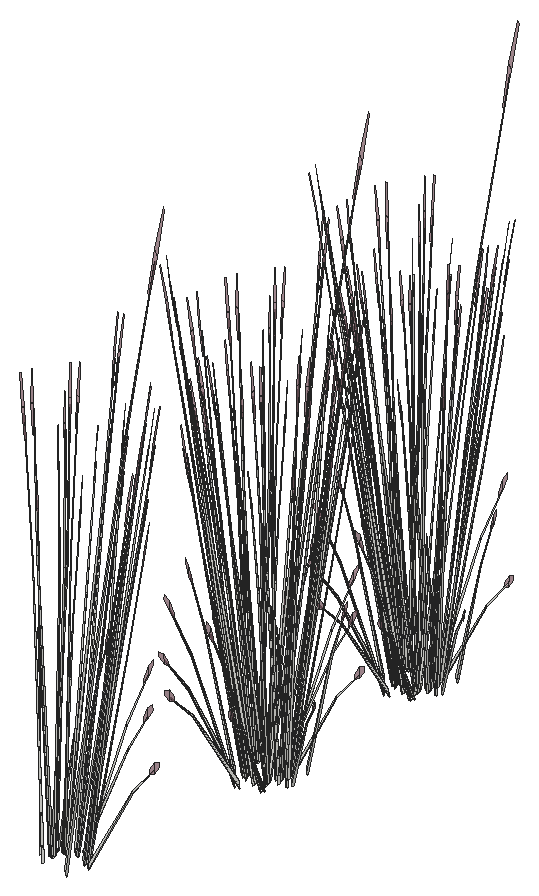
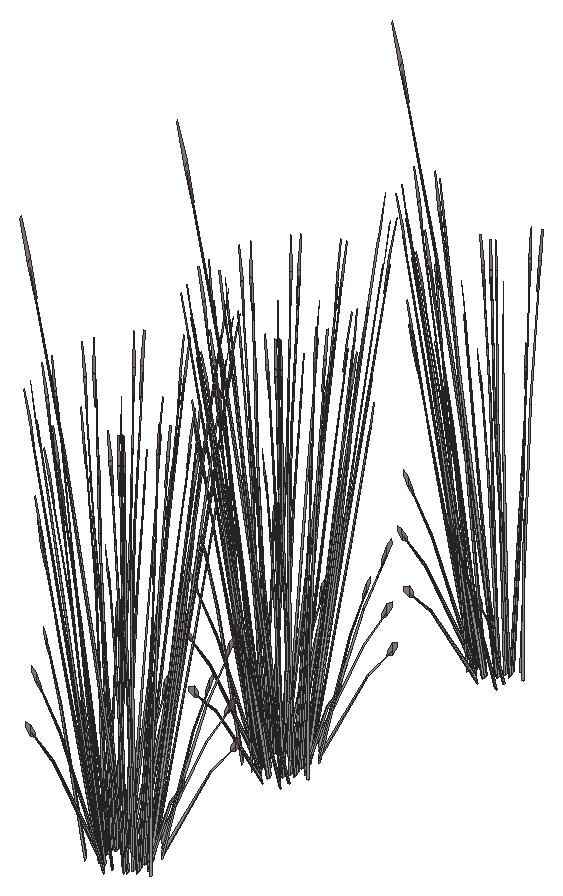
# SketchUp Ruby script. Lengths in inches.
U = 1.inch
M = Sketchup.active_model
def pt(a) = Geom::Point3d.new(a.map { |v| v * U })
def face(e, loops, mat)
  f = e.add_face(loops[0].map { |a| pt(a) })
  loops[1..].each { |l| e.add_face(l.map { |a| pt(a) }).erase! }
  f.material = f.back_material = mat if mat
  f
end
# faces: each face lists its corners as indices into pts; further lists are holes
def faces(e, pts, list, mat = nil) = list.each { |f| face(e, (f[0].is_a?(Array) ? f : [f]).map { |l| l.map { |i| pts[i] } }, mat) }
# xy, xz, yz: faces in a plane at the given z, y or x. An outline is a flat list of corners, or four numbers for a rectangle; further outlines are holes
def ring(l) = l.size == 4 ? [[l[0], l[1]], [l[2], l[1]], [l[2], l[3]], [l[0], l[3]]] : l.each_slice(2).to_a
def flat(e, list, mat, &to3) = list.each { |f| face(e, (f[0].is_a?(Array) ? f : [f]).map { |l| ring(l).map { |u, v| to3.(u, v) } }, mat) }
def xy(e, z, list, mat = nil) = flat(e, list, mat) { |x, y| [x, y, z] }
def xz(e, y, list, mat = nil) = flat(e, list, mat) { |x, z| [x, y, z] }
def yz(e, x, list, mat = nil) = flat(e, list, mat) { |y, z| [x, y, z] }
def lines(e, pts, list) = list.each { |a, b| e.add_line(pt(pts[a]), pt(pts[b])) }
# prism: a flat outline (further loops are holes) pulled along v
def prism(e, loops, v, mat = nil)
  f = face(e, loops, mat); d = Geom::Vector3d.new(v.map { |x| x * U })
  f.pushpull(f.normal.samedirection?(d) ? d.length : -d.length)
end
def box(e, o, s, mat = nil) = prism(e, [[o, [o[0] + s[0], o[1], o[2]], [o[0] + s[0], o[1] + s[1], o[2]], [o[0], o[1] + s[1], o[2]]]], [0, 0, s[2]], mat)
def at(x, y, z, deg = 0) = Geom::Transformation.translation(pt([x, y, z])) * Geom::Transformation.rotation(ORIGIN, Z_AXIS, deg.degrees)
def axes(o, x, y, z) = Geom::Transformation.new([*x, 0, *y, 0, *z, 0, *pt(o).to_a, 1])
def part(name) = M.definitions.add(name)
# library, detail: a bought-in or finely detailed component or shape, given as its bounding box
def library(name, o, s) = part(name).tap { |d| box(d.entities, o, s) }
def detail(e, o, s) = box(e.add_group.entities, o, s)
def put(e, d, t, mat = nil) = e.add_instance(d, t).tap { |i| i.material = mat if mat }
def group(e, t, mat = nil) = e.add_group.tap { |g| g.transformation = t; g.material = mat if mat }.entities
root = M.entities
M.materials.add("LightPink_Translucent").color = [144, 107, 117]
M.materials["LightPink_Translucent"].alpha = 0.75
c1 = part("blade")
p = [[2.15,0.21,22],[0,0.17,0],[0.09,0.45,0],[2.18,0.31,22],[2.29,0.31,22],[0.38,0.45,0],
  [2.48,0.24,33],[2.49,0.24,33],[2.48,0.22,33]]
faces(c1.entities,p,[[0,1,2,3],[4,5,2,3],[6,3,4,7],[8,0,3,6]])
c2 = part("seeds")
p = [[0.3,-0.1,1.38],[-0.01,-0.03,1.59],[-0.01,-0.03,0.03],[0.14,-0.07,-0.07],[0.29,-0.03,3],[0.15,0.01,3.11]]
faces(c2.entities,p,[[0,1,2,3],[1,0,4,5]],"LightPink_Translucent")
c3 = part("blade with seeds")
put(c3.entities,c1,at(0,0,0))
put(c3.entities,c2,axes([2.4,0.25,30.99],[1.5799,-0.05474,1.17369],[-0.12525,1.92788,0.29478],[-0.07173,-0.02425,1.56792]))
put(root,c3,axes([397.78,218.14,5.03],[0.17758,0.42229,-0.1216],[-0.31518,0.20752,-0.67495],[-0.13282,0.05572,1.02557]))
put(root,c3,axes([400.46,219.96,5.03],[0.0189,-0.47427,-0.1216],[0.35781,0.01296,-0.67495],[0.13781,0.03295,1.02557]))
put(root,c3,axes([400.4,219.78,5.05],[-0.20082,-0.29199,0.35414],[0.2293,-0.2764,-0.4572],[0.1165,0.04206,0.87481]))
put(root,c3,axes([400.77,219.68,4.72],[0.07571,-0.00789,1.74944],[0.20767,-0.36231,-0.27667],[0.13467,0.04783,0.14031]))
put(root,c3,axes([397.74,219.32,4.73],[-0.08753,-0.42921,0.48003],[0.34336,-0.07449,0.3958],[-0.1012,0.10094,0.9933]))
put(root,c3,axes([397.68,219.24,4.73],[-0.2423,-0.19613,0.0643],[0.14107,-0.2793,0.50621],[-0.07768,0.0903,0.77189]))
put(root,c3,axes([397.95,219.18,5.05],[0.30722,-0.06665,0.35414],[0.08112,0.381,-0.4572],[-0.08804,0.10234,0.87481]))
put(root,c3,axes([396.77,219.01,4.71],[0.04504,0.01251,1.77383],[0.13934,0.41205,-0.16761],[-0.0922,0.10815,0.31391]))
put(root,c3,axes([400.59,220.04,4.73],[-0.01777,0.35463,0.0643],[-0.26836,-0.00972,0.50621],[0.1028,0.03711,0.77189]))
put(root,c3,axes([400.61,219.93,4.73],[-0.26024,0.30729,0.48003],[-0.22444,-0.32634,0.3958],[0.1221,0.05668,0.9933]))
put(root,c3,axes([397.26,220.26,5.65],[0.31145,0.12449,-0.06488],[-0.0958,0.38314,-0.29416],[-0.05094,0.05817,0.97024]))
put(root,c3,axes([399.78,220.29,5.05],[-0.05451,-0.37564,0.35414],[0.31161,-0.09919,-0.4572],[0.0837,0.10765,0.87481]))
put(root,c3,axes([399.99,218.125,4.47],[-0.30498,-0.24231,1.38283],[0.32203,-0.37727,0.59665],[0.0984,0.22736,1.33663]))
put(root,c3,axes([397.79,219.15,5.03],[0.32648,0.25715,-0.1216],[-0.18809,0.3724,-0.67495],[-0.09224,0.12945,1.02557]))
put(root,c3,axes([399.75,220.48,5.03],[0.21031,-0.39918,-0.1216],[0.30457,0.22997,-0.67495],[0.10587,0.11278,1.02557]))
put(root,c3,axes([398.37,219.94,5.05],[0.23881,-0.24554,0.35414],[0.22606,0.28036,-0.4572],[-0.0344,0.14245,0.87481]))
put(root,c3,axes([399.48,220.8125,4.71],[0.00104,-0.05646,1.77383],[0.30246,-0.2491,-0.16761],[0.10506,0.08891,0.31391]))
put(root,c3,axes([398.15,220.16,4.73],[-0.29004,-0.02173,0.0643],[0.00795,-0.32812,0.50621],[-0.03035,0.12569,0.77189]))
put(root,c3,axes([398.24,220.19,4.73],[-0.25132,-0.3182,0.48003],[0.2669,-0.27442,0.3958],[-0.04636,0.14929,0.9933]))
put(root,c3,axes([399.04,220.35,5.05],[0.1064,-0.35863,0.35414],[0.31043,0.1046,-0.4572],[0.02846,0.14439,0.87481]))
put(root,c3,axes([399.83,220.625,4.73],[-0.16041,0.29625,0.0643],[-0.22843,-0.17248,0.50621],[0.07385,0.09498,0.77189]))
put(root,c3,axes([399.46,221.625,5.65],[0.2439,-0.26754,-0.06488],[0.22348,0.29302,-0.29416],[0.01573,0.08303,0.97024]))
put(root,c3,axes([399.9,220.54,4.73],[-0.35104,0.10702,0.48003],[-0.06092,-0.41983,0.3958],[0.08256,0.12373,0.9933]))
put(root,c3,axes([398.94,220.67,4.73],[-0.26007,0.1585,0.0643],[-0.12729,-0.28902,0.50621],[0.02512,0.1274,0.77189]))
put(root,c3,axes([397.42,220.22,4.72],[-0.00877,0.09229,1.74944],[0.24897,0.32105,-0.27667],[-0.06518,0.15182,0.14031]))
put(root,c3,axes([398.22,220.01,5.4],[0.3879,0.02311,-0.13498],[-0.0106,0.43749,-0.74919],[-0.02694,0.1685,1.13838]))
put(root,c3,axes([398.93,220.5,5.03],[0.34538,-0.21713,-0.1216],[0.16972,0.38536,-0.67495],[0.04557,0.16239,1.02557]))
put(root,c3,axes([399.03,220.64,5.0625],[-0.34777,-0.12192,0.53283],[0.11892,-0.40083,0.43934],[0.0209,0.15763,1.10256]))
put(root,c3,axes([397.39,221.16,4.71],[0.04004,-0.02816,1.77383],[0.33095,0.18728,-0.16761],[-0.00778,0.15594,0.31391]))
put(root,c3,axes([398.85,221.36,4.72],[0.04474,0.0751,1.74944],[0.36104,0.0295,-0.27667],[0.03631,0.16562,0.14031]))
put(root,c3,axes([401.89,235.44,4.72],[-0.05398,-0.06539,1.74944],[-0.36026,0.04145,-0.27667],[-0.0575,-0.15639,0.14031]))
put(root,c3,axes([403.51,236.24,4.72],[-0.00341,-0.09282,1.74944],[-0.28775,-0.26825,-0.27667],[0.04449,-0.16261,0.14031]))
put(root,c3,axes([403.43,235.91,4.71],[-0.03584,0.03562,1.77383],[-0.35118,-0.12018,-0.16761],[-0.01271,-0.15545,0.31391]))
put(root,c3,axes([401.52,235.23,4.71],[-0.00658,0.0559,1.77383],[-0.32474,0.20287,-0.16761],[-0.09556,-0.1037,0.31391]))
put(root,c3,axes([401.45,236.22,5.09],[0.39316,-0.11987,0.53763],[0.06823,0.47021,0.4433],[-0.09247,-0.13858,1.11249]))
put(root,c3,axes([402.34,236.31,4.73],[0.34777,0.12192,0.48003],[-0.11892,0.40083,0.3958],[-0.0209,-0.15763,0.9933]))
put(root,c3,axes([402.4375,236.45,5.03],[-0.34538,0.21713,-0.1216],[-0.16972,-0.38536,-0.67495],[-0.04557,-0.16239,1.02557]))
put(root,c3,axes([403.15,236.9375,5.03],[-0.3879,-0.02311,-0.1216],[0.0106,-0.43749,-0.67495],[0.02694,-0.1685,1.02557]))
put(root,c3,axes([402.43,236.28,4.73],[0.26007,-0.1585,0.0643],[0.12729,0.28902,0.50621],[-0.02512,-0.1274,0.77189]))
put(root,c3,axes([401.54,236.32,4.73],[0.16041,-0.29625,0.0643],[0.22843,0.17248,0.50621],[-0.07385,-0.09498,0.77189]))
put(root,c3,axes([402.33,236.6,5.05],[-0.1064,0.35863,0.35414],[-0.31043,-0.1046,-0.4572],[-0.02846,-0.14439,0.87481]))
put(root,c3,axes([403.125,236.75,4.73],[0.25132,0.3182,0.48003],[-0.2669,0.27442,0.3958],[0.04636,-0.14929,0.9933]))
put(root,c3,axes([401.61,236.29,5.43],[-0.23555,0.44708,-0.13619],[-0.34112,-0.25757,-0.75594],[-0.11858,-0.12631,1.14864]))
put(root,c3,axes([403.22,236.78,4.73],[0.29004,0.02173,0.0643],[-0.00795,0.32812,0.50621],[0.03035,-0.12569,0.77189]))
put(root,c3,axes([403,237.01,5.05],[-0.23881,0.24554,0.35414],[-0.22606,-0.28036,-0.4572],[0.0344,-0.14245,0.87481]))
put(root,c3,axes([400.71,236.16,4.72],[-0.07594,-0.00329,1.74944],[-0.24177,0.32918,-0.27667],[-0.129,-0.06726,0.14031]))
put(root,c3,axes([403.58,237.8,5.03],[-0.32648,-0.25715,-0.1216],[0.18809,-0.3724,-0.67495],[0.09224,-0.12945,1.02557]))
put(root,c3,axes([401.59,236.66,5.05],[0.05451,0.37564,0.35414],[-0.31161,0.09919,-0.4572],[-0.0837,-0.10765,0.87481]))
put(root,c3,axes([400.65,236.91,5.09],[0.29147,-0.34417,0.53763],[0.25138,0.3655,0.4433],[-0.13675,-0.06349,1.11249]))
put(root,c3,axes([404.38,237.6875,4.71],[-0.0461,-0.00354,1.77383],[-0.19143,-0.37951,-0.16761],[0.07688,-0.12478,0.31391]))
put(root,c3,axes([400.78,236.9,4.73],[0.01777,-0.35463,0.0643],[0.26836,0.00972,0.50621],[-0.1028,-0.03711,0.77189]))
put(root,c3,axes([403.42,237.76,5.05],[-0.30722,0.06665,0.35414],[-0.08112,-0.381,-0.4572],[0.08804,-0.10234,0.87481]))
put(root,c3,axes([403.7,237.7,4.73],[0.2423,0.19613,0.0643],[-0.14107,0.2793,0.50621],[0.07768,-0.0903,0.77189]))
put(root,c3,axes([403.63,237.62,4.73],[0.08753,0.42921,0.48003],[-0.34336,0.07449,0.3958],[0.1012,-0.10094,0.9933]))
put(root,c3,axes([404.55,238.14,4.72],[0.04898,-0.07104,1.74944],[-0.06269,-0.43574,-0.27667],[0.12289,-0.08262,0.14031]))
put(root,c3,axes([400.42,236.44,4.71],[0.02617,0.04654,1.77383],[-0.12614,0.41836,-0.16761],[-0.12775,0.00303,0.31391]))
put(root,c3,axes([400.97,237.17,5.05],[0.20082,0.29199,0.35414],[-0.2293,0.2764,-0.4572],[-0.1165,-0.04206,0.87481]))
put(root,c3,axes([400.91,236.98,5.03],[-0.0189,0.47427,-0.1216],[-0.35781,-0.01296,-0.67495],[-0.13781,-0.03295,1.02557]))
put(root,c3,axes([403.59,238.8,5.03],[-0.17758,-0.42229,-0.1216],[0.31518,-0.20752,-0.67495],[0.13282,-0.05572,1.02557]))
put(root,c3,axes([403.47,238.68,5.05],[-0.29332,-0.1301,0.35414],[0.08555,-0.37955,-0.4572],[0.11809,-0.0348,0.87481]))
put(root,c3,axes([400.4,237.98,4.73],[0.09971,-0.42522,0.48003],[0.32782,0.1454,0.3958],[-0.12892,0.02555,0.9933]))
put(root,c3,axes([400.37,237.87,4.73],[-0.12963,-0.31798,0.0643],[0.23638,-0.15564,0.50621],[-0.1042,0.03071,0.77189]))
put(root,c3,axes([403.73,238.79,4.73],[0.12963,0.31798,0.0643],[-0.23638,0.15564,0.50621],[0.1042,-0.03071,0.77189]))
put(root,c3,axes([403.71,238.68,4.73],[-0.09971,0.42522,0.48003],[-0.32782,-0.1454,0.3958],[0.12892,-0.02555,0.9933]))
put(root,c3,axes([400.64,237.99,5.05],[0.29332,0.1301,0.35414],[-0.08555,0.37955,-0.4572],[-0.11809,0.0348,0.87481]))
put(root,c3,axes([404.3,240.06,4.71],[-0.03191,-0.04083,1.77383],[0.06981,-0.43764,-0.16761],[0.12571,-0.02796,0.31391]))
put(root,c3,axes([400.14,238.28,4.72],[-0.05763,0.06055,1.74944],[0.0049,0.44239,-0.27667],[-0.13211,0.05753,0.14031]))
put(root,c3,axes([400.51,237.86,5.03],[0.17758,0.42229,-0.1216],[-0.31518,0.20752,-0.67495],[-0.13282,0.05572,1.02557]))
put(root,c3,axes([403.19,239.68,5.03],[0.0189,-0.47427,-0.1216],[0.35781,0.01296,-0.67495],[0.13781,0.03295,1.02557]))
put(root,c3,axes([403.14,239.49,5.05],[-0.20082,-0.29199,0.35414],[0.2293,-0.2764,-0.4572],[0.1165,0.04206,0.87481]))
put(root,c3,axes([403.5,239.4,4.72],[0.07571,-0.00789,1.74944],[0.20767,-0.36231,-0.27667],[0.13467,0.04783,0.14031]))
put(root,c3,axes([400.47,239.04,4.73],[-0.08753,-0.42921,0.48003],[0.34336,-0.07449,0.3958],[-0.1012,0.10094,0.9933]))
put(root,c3,axes([400.41,238.96,4.73],[-0.2423,-0.19613,0.0643],[0.14107,-0.2793,0.50621],[-0.07768,0.0903,0.77189]))
put(root,c3,axes([400.6875,238.9,5.05],[0.30722,-0.06665,0.35414],[0.08112,0.381,-0.4572],[-0.08804,0.10234,0.87481]))
put(root,c3,axes([399.5,238.73,4.71],[0.04504,0.01251,1.77383],[0.13934,0.41205,-0.16761],[-0.0922,0.10815,0.31391]))
put(root,c3,axes([403.32,239.76,4.73],[-0.01777,0.35463,0.0643],[-0.26836,-0.00972,0.50621],[0.1028,0.03711,0.77189]))
put(root,c3,axes([403.34,239.65,4.73],[-0.26024,0.30729,0.48003],[-0.22444,-0.32634,0.3958],[0.1221,0.05668,0.9933]))
put(root,c3,axes([399.99,239.98,5.65],[0.31145,0.12449,-0.06488],[-0.0958,0.38314,-0.29416],[-0.05094,0.05817,0.97024]))
put(root,c3,axes([402.52,240,5.05],[-0.05451,-0.37564,0.35414],[0.31161,-0.09919,-0.4572],[0.0837,0.10765,0.87481]))
put(root,c3,axes([402.72,237.84,4.47],[-0.30498,-0.24231,1.38283],[0.32203,-0.37727,0.59665],[0.0984,0.22736,1.33663]))
put(root,c3,axes([400.53,238.86,5.03],[0.32648,0.25715,-0.1216],[-0.18809,0.3724,-0.67495],[-0.09224,0.12945,1.02557]))
put(root,c3,axes([402.49,240.2,5.03],[0.21031,-0.39918,-0.1216],[0.30457,0.22997,-0.67495],[0.10587,0.11278,1.02557]))
put(root,c3,axes([401.1,239.66,5.05],[0.23881,-0.24554,0.35414],[0.22606,0.28036,-0.4572],[-0.0344,0.14245,0.87481]))
put(root,c3,axes([402.21,240.53,4.71],[0.00104,-0.05646,1.77383],[0.30246,-0.2491,-0.16761],[0.10506,0.08891,0.31391]))
put(root,c3,axes([400.88,239.88,4.73],[-0.29004,-0.02173,0.0643],[0.00795,-0.32812,0.50621],[-0.03035,0.12569,0.77189]))
put(root,c3,axes([400.98,239.91,4.73],[-0.25132,-0.3182,0.48003],[0.2669,-0.27442,0.3958],[-0.04636,0.14929,0.9933]))
put(root,c3,axes([401.77,240.0625,5.05],[0.1064,-0.35863,0.35414],[0.31043,0.1046,-0.4572],[0.02846,0.14439,0.87481]))
put(root,c3,axes([402.56,240.34,4.73],[-0.16041,0.29625,0.0643],[-0.22843,-0.17248,0.50621],[0.07385,0.09498,0.77189]))
put(root,c3,axes([402.1875,241.34,5.65],[0.2439,-0.26754,-0.06488],[0.22348,0.29302,-0.29416],[0.01573,0.08303,0.97024]))
put(root,c3,axes([402.63,240.26,4.73],[-0.35104,0.10702,0.48003],[-0.06092,-0.41983,0.3958],[0.08256,0.12373,0.9933]))
put(root,c3,axes([401.67,240.39,4.73],[-0.26007,0.1585,0.0643],[-0.12729,-0.28902,0.50621],[0.02512,0.1274,0.77189]))
put(root,c3,axes([400.15,239.93,4.72],[-0.00877,0.09229,1.74944],[0.24897,0.32105,-0.27667],[-0.06518,0.15182,0.14031]))
put(root,c3,axes([400.95,239.72,5.4],[0.3879,0.02311,-0.13498],[-0.0106,0.43749,-0.74919],[-0.02694,0.1685,1.13838]))
put(root,c3,axes([401.67,240.21,5.03],[0.34538,-0.21713,-0.1216],[0.16972,0.38536,-0.67495],[0.04557,0.16239,1.02557]))
put(root,c3,axes([401.77,240.36,5.0625],[-0.34777,-0.12192,0.53283],[0.11892,-0.40083,0.43934],[0.0209,0.15763,1.10256]))
put(root,c3,axes([400.125,240.88,4.71],[0.04004,-0.02816,1.77383],[0.33095,0.18728,-0.16761],[-0.00778,0.15594,0.31391]))
put(root,c3,axes([401.58,241.07,4.72],[0.04474,0.0751,1.74944],[0.36104,0.0295,-0.27667],[0.03631,0.16562,0.14031]))
put(root,c3,axes([401.89,252.32,4.72],[-0.05398,-0.06539,1.74944],[-0.36026,0.04145,-0.27667],[-0.0575,-0.15639,0.14031]))
put(root,c3,axes([403.51,253.12,4.72],[-0.00341,-0.09282,1.74944],[-0.28775,-0.26825,-0.27667],[0.04449,-0.16261,0.14031]))
put(root,c3,axes([403.43,252.79,4.71],[-0.03584,0.03562,1.77383],[-0.35118,-0.12018,-0.16761],[-0.01271,-0.15545,0.31391]))
put(root,c3,axes([401.52,252.11,4.71],[-0.00658,0.0559,1.77383],[-0.32474,0.20287,-0.16761],[-0.09556,-0.1037,0.31391]))
put(root,c3,axes([401.45,253.1,5.09],[0.39316,-0.11987,0.53763],[0.06823,0.47021,0.4433],[-0.09247,-0.13858,1.11249]))
put(root,c3,axes([402.34,253.1875,4.73],[0.34777,0.12192,0.48003],[-0.11892,0.40083,0.3958],[-0.0209,-0.15763,0.9933]))
put(root,c3,axes([402.4375,253.33,5.03],[-0.34538,0.21713,-0.1216],[-0.16972,-0.38536,-0.67495],[-0.04557,-0.16239,1.02557]))
put(root,c3,axes([403.15,253.82,5.03],[-0.3879,-0.02311,-0.1216],[0.0106,-0.43749,-0.67495],[0.02694,-0.1685,1.02557]))
put(root,c3,axes([402.43,253.16,4.73],[0.26007,-0.1585,0.0643],[0.12729,0.28902,0.50621],[-0.02512,-0.1274,0.77189]))
put(root,c3,axes([401.54,253.2,4.73],[0.16041,-0.29625,0.0643],[0.22843,0.17248,0.50621],[-0.07385,-0.09498,0.77189]))
put(root,c3,axes([402.33,253.48,5.05],[-0.1064,0.35863,0.35414],[-0.31043,-0.1046,-0.4572],[-0.02846,-0.14439,0.87481]))
put(root,c3,axes([403.125,253.63,4.73],[0.25132,0.3182,0.48003],[-0.2669,0.27442,0.3958],[0.04636,-0.14929,0.9933]))
put(root,c3,axes([401.61,253.17,5.43],[-0.23555,0.44708,-0.13619],[-0.34112,-0.25757,-0.75594],[-0.11858,-0.12631,1.14864]))
put(root,c3,axes([403.22,253.66,4.73],[0.29004,0.02173,0.0643],[-0.00795,0.32812,0.50621],[0.03035,-0.12569,0.77189]))
put(root,c3,axes([403,253.88,5.05],[-0.23881,0.24554,0.35414],[-0.22606,-0.28036,-0.4572],[0.0344,-0.14245,0.87481]))
put(root,c3,axes([400.71,253.04,4.72],[-0.07594,-0.00329,1.74944],[-0.24177,0.32918,-0.27667],[-0.129,-0.06726,0.14031]))
put(root,c3,axes([403.58,254.68,5.03],[-0.32648,-0.25715,-0.1216],[0.18809,-0.3724,-0.67495],[0.09224,-0.12945,1.02557]))
put(root,c3,axes([401.59,253.54,5.05],[0.05451,0.37564,0.35414],[-0.31161,0.09919,-0.4572],[-0.0837,-0.10765,0.87481]))
put(root,c3,axes([400.65,253.78,5.09],[0.29147,-0.34417,0.53763],[0.25138,0.3655,0.4433],[-0.13675,-0.06349,1.11249]))
put(root,c3,axes([404.38,254.57,4.71],[-0.0461,-0.00354,1.77383],[-0.19143,-0.37951,-0.16761],[0.07688,-0.12478,0.31391]))
put(root,c3,axes([400.78,253.78,4.73],[0.01777,-0.35463,0.0643],[0.26836,0.00972,0.50621],[-0.1028,-0.03711,0.77189]))
put(root,c3,axes([403.42,254.64,5.05],[-0.30722,0.06665,0.35414],[-0.08112,-0.381,-0.4572],[0.08804,-0.10234,0.87481]))
put(root,c3,axes([403.7,254.58,4.73],[0.2423,0.19613,0.0643],[-0.14107,0.2793,0.50621],[0.07768,-0.0903,0.77189]))
put(root,c3,axes([403.63,254.5,4.73],[0.08753,0.42921,0.48003],[-0.34336,0.07449,0.3958],[0.1012,-0.10094,0.9933]))
put(root,c3,axes([404.55,255.02,4.72],[0.04898,-0.07104,1.74944],[-0.06269,-0.43574,-0.27667],[0.12289,-0.08262,0.14031]))
put(root,c3,axes([400.42,253.32,4.71],[0.02617,0.04654,1.77383],[-0.12614,0.41836,-0.16761],[-0.12775,0.00303,0.31391]))
put(root,c3,axes([400.97,254.05,5.05],[0.20082,0.29199,0.35414],[-0.2293,0.2764,-0.4572],[-0.1165,-0.04206,0.87481]))
put(root,c3,axes([400.91,253.86,5.03],[-0.0189,0.47427,-0.1216],[-0.35781,-0.01296,-0.67495],[-0.13781,-0.03295,1.02557]))
put(root,c3,axes([403.59,255.68,5.03],[-0.17758,-0.42229,-0.1216],[0.31518,-0.20752,-0.67495],[0.13282,-0.05572,1.02557]))
put(root,c3,axes([403.47,255.55,5.05],[-0.29332,-0.1301,0.35414],[0.08555,-0.37955,-0.4572],[0.11809,-0.0348,0.87481]))
put(root,c3,axes([400.4,254.86,4.73],[0.09971,-0.42522,0.48003],[0.32782,0.1454,0.3958],[-0.12892,0.02555,0.9933]))
put(root,c3,axes([400.37,254.75,4.73],[-0.12963,-0.31798,0.0643],[0.23638,-0.15564,0.50621],[-0.1042,0.03071,0.77189]))
put(root,c3,axes([403.73,255.67,4.73],[0.12963,0.31798,0.0643],[-0.23638,0.15564,0.50621],[0.1042,-0.03071,0.77189]))
put(root,c3,axes([403.71,255.56,4.73],[-0.09971,0.42522,0.48003],[-0.32782,-0.1454,0.3958],[0.12892,-0.02555,0.9933]))
put(root,c3,axes([400.64,254.87,5.05],[0.29332,0.1301,0.35414],[-0.08555,0.37955,-0.4572],[-0.11809,0.0348,0.87481]))
put(root,c3,axes([404.3,256.9375,4.71],[-0.03191,-0.04083,1.77383],[0.06981,-0.43764,-0.16761],[0.12571,-0.02796,0.31391]))
put(root,c3,axes([400.14,255.16,4.72],[-0.05763,0.06055,1.74944],[0.0049,0.44239,-0.27667],[-0.13211,0.05753,0.14031]))
put(root,c3,axes([400.51,254.74,5.03],[0.17758,0.42229,-0.1216],[-0.31518,0.20752,-0.67495],[-0.13282,0.05572,1.02557]))
put(root,c3,axes([403.19,256.56,5.03],[0.0189,-0.47427,-0.1216],[0.35781,0.01296,-0.67495],[0.13781,0.03295,1.02557]))
put(root,c3,axes([403.14,256.375,5.05],[-0.20082,-0.29199,0.35414],[0.2293,-0.2764,-0.4572],[0.1165,0.04206,0.87481]))
put(root,c3,axes([403.5,256.27,4.72],[0.07571,-0.00789,1.74944],[0.20767,-0.36231,-0.27667],[0.13467,0.04783,0.14031]))
put(root,c3,axes([400.47,255.92,4.73],[-0.08753,-0.42921,0.48003],[0.34336,-0.07449,0.3958],[-0.1012,0.10094,0.9933]))
put(root,c3,axes([400.41,255.84,4.73],[-0.2423,-0.19613,0.0643],[0.14107,-0.2793,0.50621],[-0.07768,0.0903,0.77189]))
put(root,c3,axes([400.6875,255.78,5.05],[0.30722,-0.06665,0.35414],[0.08112,0.381,-0.4572],[-0.08804,0.10234,0.87481]))
put(root,c3,axes([399.5,255.61,4.71],[0.04504,0.01251,1.77383],[0.13934,0.41205,-0.16761],[-0.0922,0.10815,0.31391]))
put(root,c3,axes([403.32,256.64,4.73],[-0.01777,0.35463,0.0643],[-0.26836,-0.00972,0.50621],[0.1028,0.03711,0.77189]))
put(root,c3,axes([403.34,256.52,4.73],[-0.26024,0.30729,0.48003],[-0.22444,-0.32634,0.3958],[0.1221,0.05668,0.9933]))
put(root,c3,axes([399.99,256.86,5.65],[0.31145,0.12449,-0.06488],[-0.0958,0.38314,-0.29416],[-0.05094,0.05817,0.97024]))
put(root,c3,axes([402.52,256.88,5.05],[-0.05451,-0.37564,0.35414],[0.31161,-0.09919,-0.4572],[0.0837,0.10765,0.87481]))
put(root,c3,axes([402.72,254.72,4.47],[-0.30498,-0.24231,1.38283],[0.32203,-0.37727,0.59665],[0.0984,0.22736,1.33663]))
put(root,c3,axes([400.53,255.74,5.03],[0.32648,0.25715,-0.1216],[-0.18809,0.3724,-0.67495],[-0.09224,0.12945,1.02557]))
put(root,c3,axes([402.49,257.07,5.03],[0.21031,-0.39918,-0.1216],[0.30457,0.22997,-0.67495],[0.10587,0.11278,1.02557]))
put(root,c3,axes([401.1,256.54,5.05],[0.23881,-0.24554,0.35414],[0.22606,0.28036,-0.4572],[-0.0344,0.14245,0.87481]))
put(root,c3,axes([402.21,257.41,4.71],[0.00104,-0.05646,1.77383],[0.30246,-0.2491,-0.16761],[0.10506,0.08891,0.31391]))
put(root,c3,axes([400.88,256.76,4.73],[-0.29004,-0.02173,0.0643],[0.00795,-0.32812,0.50621],[-0.03035,0.12569,0.77189]))
put(root,c3,axes([400.98,256.79,4.73],[-0.25132,-0.3182,0.48003],[0.2669,-0.27442,0.3958],[-0.04636,0.14929,0.9933]))
put(root,c3,axes([401.77,256.94,5.05],[0.1064,-0.35863,0.35414],[0.31043,0.1046,-0.4572],[0.02846,0.14439,0.87481]))
put(root,c3,axes([402.56,257.22,4.73],[-0.16041,0.29625,0.0643],[-0.22843,-0.17248,0.50621],[0.07385,0.09498,0.77189]))
